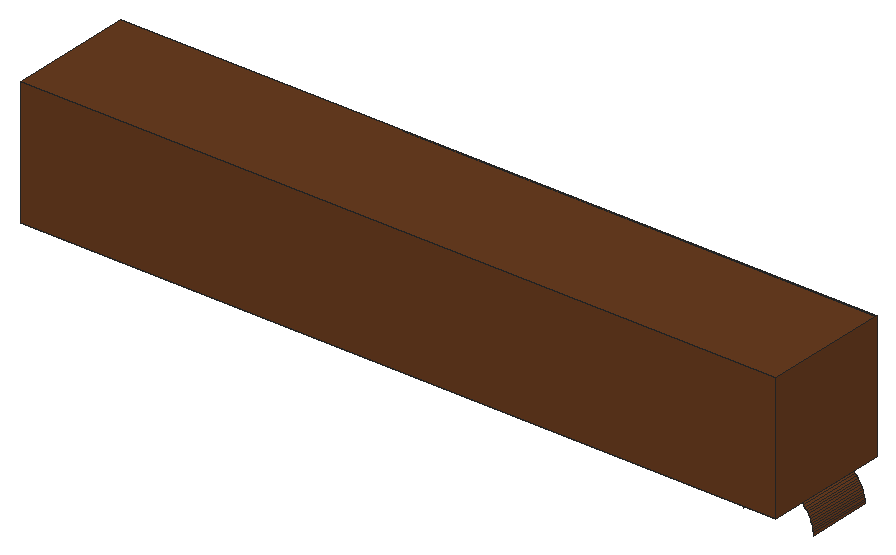
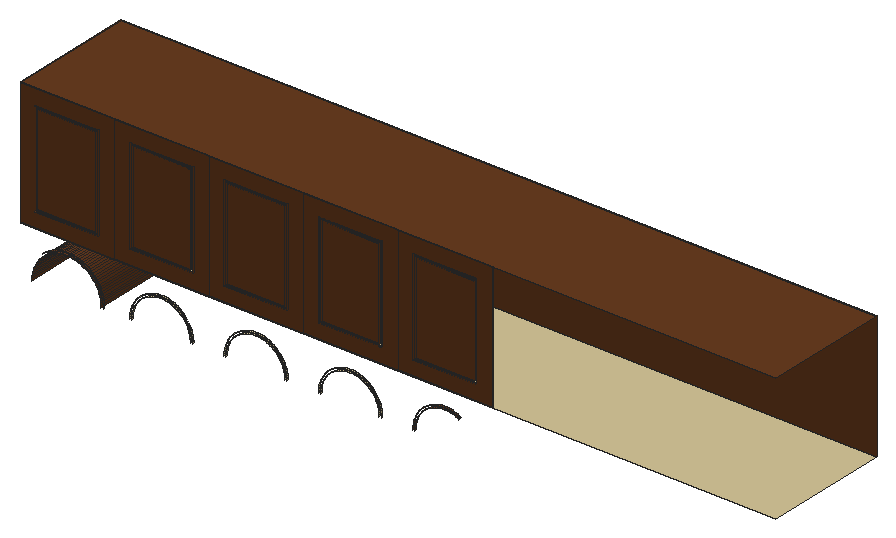
# SketchUp Ruby script. Lengths in inches.
U = 1.inch
M = Sketchup.active_model
def pt(a) = Geom::Point3d.new(a.map { |v| v * U })
def face(e, loops, mat)
  f = e.add_face(loops[0].map { |a| pt(a) })
  loops[1..].each { |l| e.add_face(l.map { |a| pt(a) }).erase! }
  f.material = f.back_material = mat if mat
  f
end
# faces: each face lists its corners as indices into pts; further lists are holes
def faces(e, pts, list, mat = nil) = list.each { |f| face(e, (f[0].is_a?(Array) ? f : [f]).map { |l| l.map { |i| pts[i] } }, mat) }
# xy, xz, yz: faces in a plane at the given z, y or x. An outline is a flat list of corners, or four numbers for a rectangle; further outlines are holes
def ring(l) = l.size == 4 ? [[l[0], l[1]], [l[2], l[1]], [l[2], l[3]], [l[0], l[3]]] : l.each_slice(2).to_a
def flat(e, list, mat, &to3) = list.each { |f| face(e, (f[0].is_a?(Array) ? f : [f]).map { |l| ring(l).map { |u, v| to3.(u, v) } }, mat) }
def xy(e, z, list, mat = nil) = flat(e, list, mat) { |x, y| [x, y, z] }
def xz(e, y, list, mat = nil) = flat(e, list, mat) { |x, z| [x, y, z] }
def yz(e, x, list, mat = nil) = flat(e, list, mat) { |y, z| [x, y, z] }
def lines(e, pts, list) = list.each { |a, b| e.add_line(pt(pts[a]), pt(pts[b])) }
# prism: a flat outline (further loops are holes) pulled along v
def prism(e, loops, v, mat = nil)
  f = face(e, loops, mat); d = Geom::Vector3d.new(v.map { |x| x * U })
  f.pushpull(f.normal.samedirection?(d) ? d.length : -d.length)
end
def box(e, o, s, mat = nil) = prism(e, [[o, [o[0] + s[0], o[1], o[2]], [o[0] + s[0], o[1] + s[1], o[2]], [o[0], o[1] + s[1], o[2]]]], [0, 0, s[2]], mat)
def at(x, y, z, deg = 0) = Geom::Transformation.translation(pt([x, y, z])) * Geom::Transformation.rotation(ORIGIN, Z_AXIS, deg.degrees)
def axes(o, x, y, z) = Geom::Transformation.new([*x, 0, *y, 0, *z, 0, *pt(o).to_a, 1])
def part(name) = M.definitions.add(name)
# library, detail: a bought-in or finely detailed component or shape, given as its bounding box
def library(name, o, s) = part(name).tap { |d| box(d.entities, o, s) }
def detail(e, o, s) = box(e.add_group.entities, o, s)
def put(e, d, t, mat = nil) = e.add_instance(d, t).tap { |i| i.material = mat if mat }
def group(e, t, mat = nil) = e.add_group.tap { |g| g.transformation = t; g.material = mat if mat }.entities
root = M.entities
M.materials.add("138_plaster painted wall texture-seamless").color = [214, 198, 153]
M.materials.add("[0137_Black]").color = [0, 0, 0]
M.materials.add("[Wood Veneer 01]").color = [104, 60, 32]
xy(root,88,[[24,0,168,24]],"138_plaster painted wall texture-seamless")
xy(root,91,[[81,24,93,24.2],[99,24,111,24.2],[117,24,129,24.2],[135,24,147,24.2],[153,24,165,24.2]],"[Wood Veneer 01]")
xy(root,91.4,[[81.4,24,92.6,24.2],[99.4,24,110.6,24.2],[117.4,24,128.6,24.2],[135.4,24,146.6,24.2],[153.4,24,164.6,24.2]],"[Wood Veneer 01]")
xy(root,108.6,[[81.4,24,92.6,24.2],[99.4,24,110.6,24.2],[117.4,24,128.6,24.2],[135.4,24,146.6,24.2],[153.4,24,164.6,24.2]],"[Wood Veneer 01]")
xy(root,109,[[81,24,93,24.2],[99,24,111,24.2],[117,24,129,24.2],[135,24,147,24.2],[153,24,165,24.2]],"[Wood Veneer 01]")
xy(root,112,[[24,0,168,24]],"[Wood Veneer 01]")
xz(root,0,[[24,88,168,112]],"[Wood Veneer 01]")
xz(root,24,[[[78,88,96,112],[78.1,88.1,95.9,111.9]],[[96,88,114,112],[96.1,88.1,113.9,111.9]],[[114,88,132,112],[114.1,88.1,131.9,111.9]],[[132,88,150,112],[132.1,88.1,149.9,111.9]],[[150,88,168,112],[150.1,88.1,167.9,111.9]]],"[0137_Black]")
xz(root,24,[[[78.1,88.1,95.9,111.9],[81,91,93,109]],[[96.1,88.1,113.9,111.9],[99,91,111,109]],[[114.1,88.1,131.9,111.9],[117,91,129,109]],[[132.1,88.1,149.9,111.9],[135,91,147,109]],[[150.1,88.1,167.9,111.9],[153,91,165,109]],
  [81.4,91.4,92.6,108.6],[99.4,91.4,110.6,108.6],[117.4,91.4,128.6,108.6],[135.4,91.4,146.6,108.6],[153.4,91.4,164.6,108.6]],"[Wood Veneer 01]")
yz(root,92.6,[[24,91.4,24.2,108.6]],"[Wood Veneer 01]")
yz(root,93,[[24,91,24.2,109]],"[Wood Veneer 01]")
yz(root,99,[[24,91,24.2,109]],"[Wood Veneer 01]")
yz(root,99.4,[[24,91.4,24.2,108.6]],"[Wood Veneer 01]")
yz(root,110.6,[[24,91.4,24.2,108.6]],"[Wood Veneer 01]")
yz(root,111,[[24,91,24.2,109]],"[Wood Veneer 01]")
yz(root,117,[[24,91,24.2,109]],"[Wood Veneer 01]")
yz(root,117.4,[[24,91.4,24.2,108.6]],"[Wood Veneer 01]")
yz(root,128.6,[[24,91.4,24.2,108.6]],"[Wood Veneer 01]")
yz(root,129,[[24,91,24.2,109]],"[Wood Veneer 01]")
yz(root,135,[[24,91,24.2,109]],"[Wood Veneer 01]")
yz(root,135.4,[[24,91.4,24.2,108.6]],"[Wood Veneer 01]")
yz(root,146.6,[[24,91.4,24.2,108.6]],"[Wood Veneer 01]")
yz(root,147,[[24,91,24.2,109]],"[Wood Veneer 01]")
yz(root,153,[[24,91,24.2,109]],"[Wood Veneer 01]")
yz(root,153.4,[[24,91.4,24.2,108.6]],"[Wood Veneer 01]")
yz(root,168,[[0,88,24,112]],"[Wood Veneer 01]")
p = [[152.4,12,79],[152.4,24.2,79],[152.41,24.2,79.38],[152.41,12,79.38],[165.59,12,79.38],[165.59,24.2,79.38],
  [165.6,24.2,79],[165.6,12,79],[92.6,24,79],[92.59,24,79.33],[92.59,24.2,79.33],[92.6,24.2,79],
  [92.99,24,79.35],[93,24,79],[93,24.2,79],[92.99,24.2,79.35],[99,24,79],[99.01,24,79.35],
  [99.01,24.2,79.35],[99,24.2,79],[99.41,24,79.33],[99.4,24,79],[99.4,24.2,79],[99.41,24.2,79.33],
  [110.6,24,79],[110.59,24,79.33],[110.59,24.2,79.33],[110.6,24.2,79],[110.99,24,79.35],[111,24,79],
  [111,24.2,79],[110.99,24.2,79.35],[117,24,79],[117.01,24,79.35],[117.01,24.2,79.35],[117,24.2,79],
  [117.41,24,79.33],[117.4,24,79],[117.4,24.2,79],[117.41,24.2,79.33],[128.6,24,79],[128.59,24,79.33],
  [128.59,24.2,79.33],[128.6,24.2,79],[128.99,24,79.35],[129,24,79],[129,24.2,79],[128.99,24.2,79.35],
  [135,24,79],[135.01,24,79.35],[135.01,24.2,79.35],[135,24.2,79],[135.41,24,79.33],[135.4,24,79],
  [135.4,24.2,79],[135.41,24.2,79.33],[146.6,24,79],[146.59,24,79.33],[146.59,24.2,79.33],[146.6,24.2,79],
  [146.99,24,79.35],[147,24,79],[147,24.2,79],[146.99,24.2,79.35],[152,24,79],[152.01,24,79.41],
  [152.01,24.2,79.41],[152,24.2,79],[92.5625,24,79.65],[92.5625,24.2,79.65],[92.96,24,79.7],[92.96,24.2,79.7],
  [99.04,24,79.7],[99.04,24.2,79.7],[99.4375,24,79.65],[99.4375,24.2,79.65],[110.5625,24,79.65],[110.5625,24.2,79.65],
  [110.96,24,79.7],[110.96,24.2,79.7],[117.04,24,79.7],[117.04,24.2,79.7],[117.4375,24,79.65],[117.4375,24.2,79.65],
  [128.5625,24,79.65],[128.5625,24.2,79.65],[128.96,24,79.7],[128.96,24.2,79.7],[135.04,24,79.7],[135.04,24.2,79.7],
  [135.4375,24,79.65],[135.4375,24.2,79.65],[146.5625,24,79.65],[146.5625,24.2,79.65],[146.96,24,79.7],[146.96,24.2,79.7],
  [152.44,24.2,79.77],[152.44,12,79.77],[165.56,12,79.77],[165.56,24.2,79.77],[152.05,24,79.8125],[152.05,24.2,79.8125],
  [92.51,24,79.97],[92.51,24.2,79.97],[92.91,24,80.04],[92.91,24.2,80.04],[99.09,24,80.04],[99.09,24.2,80.04],
  [99.49,24,79.97],[99.49,24.2,79.97],[110.51,24,79.97],[110.51,24.2,79.97],[110.91,24,80.04],[110.91,24.2,80.04],
  [117.09,24,80.04],[117.09,24.2,80.04],[117.49,24,79.97],[117.49,24.2,79.97],[128.51,24,79.97],[128.51,24.2,79.97],
  [128.91,24,80.04],[128.91,24.2,80.04],[135.09,24,80.04],[135.09,24.2,80.04],[135.49,24,79.97],[135.49,24.2,79.97],
  [146.51,24,79.97],[146.51,24.2,79.97],[146.91,24,80.04],[146.91,24.2,80.04],[152.5,24.2,80.15],[152.5,12,80.15],
  [165.5,12,80.15],[165.5,24.2,80.15],[152.11,24,80.22],[152.11,24.2,80.22],[92.45,24,80.29],[92.45,24.2,80.29],
  [92.84,24,80.38],[92.84,24.2,80.38],[99.16,24,80.38],[99.16,24.2,80.38],[99.55,24,80.29],[99.55,24.2,80.29],
  [110.45,24,80.29],[110.45,24.2,80.29],[110.84,24,80.38],[110.84,24.2,80.38],[117.16,24,80.38],[117.16,24.2,80.38],
  [117.55,24,80.29],[117.55,24.2,80.29],[128.45,24,80.29],[128.45,24.2,80.29],[128.84,24,80.38],[128.84,24.2,80.38],
  [135.16,24,80.38],[135.16,24.2,80.38],[135.55,24,80.29],[135.55,24.2,80.29],[146.45,24,80.29],[146.45,24.2,80.29],
  [146.84,24,80.38],[146.84,24.2,80.38],[152.58,24.2,80.52],[152.58,12,80.52],[165.42,12,80.52],[165.42,24.2,80.52],
  [152.1875,24,80.61],[152.1875,24.2,80.61],[92.36,24,80.61],[92.36,24.2,80.61],[99.64,24,80.61],[99.64,24.2,80.61],
  [110.36,24,80.61],[110.36,24.2,80.61],[117.64,24,80.61],[117.64,24.2,80.61],[128.36,24,80.61],[128.36,24.2,80.61],
  [135.64,24,80.61],[135.64,24.2,80.61],[146.36,24,80.61],[146.36,24.2,80.61],[92.75,24,80.72],[92.75,24.2,80.72],
  [99.25,24,80.72],[99.25,24.2,80.72],[110.75,24,80.72],[110.75,24.2,80.72],[117.25,24,80.72],[117.25,24.2,80.72],
  [128.75,24,80.72],[128.75,24.2,80.72],[135.25,24,80.72],[135.25,24.2,80.72],[146.75,24,80.72],[146.75,24.2,80.72],
  [152.68,24.2,80.89],[152.68,12,80.89],[165.32,12,80.89],[165.32,24.2,80.89],[92.26,24,80.92],[92.26,24.2,80.92],
  [99.74,24,80.92],[99.74,24.2,80.92],[110.26,24,80.92],[110.26,24.2,80.92],[117.74,24,80.92],[117.74,24.2,80.92],
  [128.26,24,80.92],[128.26,24.2,80.92],[135.74,24,80.92],[135.74,24.2,80.92],[146.26,24,80.92],[146.26,24.2,80.92],
  [152.29,24,81.01],[152.29,24.2,81.01],[92.64,24,81.05],[92.64,24.2,81.05],[99.36,24,81.05],[99.36,24.2,81.05],
  [110.64,24,81.05],[110.64,24.2,81.05],[117.36,24,81.05],[117.36,24.2,81.05],[128.64,24,81.05],[128.64,24.2,81.05],
  [135.36,24,81.05],[135.36,24.2,81.05],[146.64,24,81.05],[146.64,24.2,81.05],[152.8,24.2,81.26],[152.8,12,81.26],
  [165.2,12,81.26],[165.2,24.2,81.26],[92.14,24,81.22],[92.14,24.2,81.22],[99.86,24,81.22],[99.86,24.2,81.22],
  [110.14,24,81.22],[110.14,24.2,81.22],[117.86,24,81.22],[117.86,24.2,81.22],[128.14,24,81.22],[128.14,24.2,81.22],
  [135.86,24,81.22],[135.86,24.2,81.22],[146.14,24,81.22],[146.14,24.2,81.22],[152.42,24,81.39],[152.42,24.2,81.39],
  [92.51,24,81.375],[92.51,24.2,81.375],[99.49,24,81.375],[99.49,24.2,81.375],[110.51,24,81.375],[110.51,24.2,81.375],
  [117.49,24,81.375],[117.49,24.2,81.375],[128.51,24,81.375],[128.51,24.2,81.375],[135.49,24,81.375],[135.49,24.2,81.375],
  [146.51,24,81.375],[146.51,24.2,81.375],[92,24,81.51],[92,24.2,81.51],[100,24,81.51],[100,24.2,81.51],
  [110,24,81.51],[110,24.2,81.51],[118,24,81.51],[118,24.2,81.51],[128,24,81.51],[128,24.2,81.51],
  [136,24,81.51],[136,24.2,81.51],[146,24,81.51],[146,24.2,81.51],[152.94,24.2,81.61],[152.94,12,81.61],
  [165.06,12,81.61],[165.06,24.2,81.61],[92.36,24,81.69],[92.36,24.2,81.69],[99.64,24,81.69],[99.64,24.2,81.69],
  [110.36,24,81.69],[110.36,24.2,81.69],[117.64,24,81.69],[117.64,24.2,81.69],[128.36,24,81.69],[128.36,24.2,81.69],
  [135.64,24,81.69],[135.64,24.2,81.69],[146.36,24,81.69],[146.36,24.2,81.69],[152.57,24,81.77],[152.57,24.2,81.77],
  [91.85,24,81.8],[91.85,24.2,81.8],[100.15,24,81.8],[100.15,24.2,81.8],[109.85,24,81.8],[109.85,24.2,81.8],
  [118.15,24,81.8],[118.15,24.2,81.8],[127.85,24,81.8],[127.85,24.2,81.8],[136.15,24,81.8],[136.15,24.2,81.8],
  [145.85,24,81.8],[145.85,24.2,81.8],[153.1,24.2,81.96],[153.1,12,81.96],[164.9,12,81.96],[164.9,24.2,81.96],
  [92.2,24,82],[92.2,24.2,82],[99.8,24,82],[99.8,24.2,82],[110.2,24,82],[110.2,24.2,82],
  [117.8,24,82],[117.8,24.2,82],[128.2,24,82],[128.2,24.2,82],[135.8,24,82],[135.8,24.2,82],
  [146.2,24,82],[146.2,24.2,82],[91.68,24,82.08],[91.68,24.2,82.08],[100.32,24,82.08],[100.32,24.2,82.08],
  [109.68,24,82.08],[109.68,24.2,82.08],[118.32,24,82.08],[118.32,24.2,82.08],[127.68,24,82.08],[127.68,24.2,82.08],
  [136.32,24,82.08],[136.32,24.2,82.08],[145.68,24,82.08],[145.68,24.2,82.08],[152.74,24,82.14],[152.74,24.2,82.14],
  [153.28,24.2,82.3],[153.28,12,82.3],[164.72,12,82.3],[164.72,24.2,82.3],[92.01,24,82.3],[92.01,24.2,82.3],
  [99.99,24,82.3],[99.99,24.2,82.3],[110.01,24,82.3],[110.01,24.2,82.3],[117.99,24,82.3],[117.99,24.2,82.3],
  [128.01,24,82.3],[128.01,24.2,82.3],[135.99,24,82.3],[135.99,24.2,82.3],[146.01,24,82.3],[146.01,24.2,82.3],
  [91.49,24,82.34],[91.49,24.2,82.34],[100.51,24,82.34],[100.51,24.2,82.34],[109.49,24,82.34],[109.49,24.2,82.34],
  [118.51,24,82.34],[118.51,24.2,82.34],[127.49,24,82.34],[127.49,24.2,82.34],[136.51,24,82.34],[136.51,24.2,82.34],
  [145.49,24,82.34],[145.49,24.2,82.34],[152.9375,24,82.5],[152.9375,24.2,82.5],[153.49,24.2,82.625],[153.49,12,82.625],
  [164.51,12,82.625],[164.51,24.2,82.625],[91.29,24,82.6],[91.29,24.2,82.6],[91.8125,24,82.58],[91.8125,24.2,82.58],
  [100.1875,24,82.58],[100.1875,24.2,82.58],[100.71,24,82.6],[100.71,24.2,82.6],[109.29,24,82.6],[109.29,24.2,82.6],
  [109.8125,24,82.58],[109.8125,24.2,82.58],[118.1875,24,82.58],[118.1875,24.2,82.58],[118.71,24,82.6],[118.71,24.2,82.6],
  [127.29,24,82.6],[127.29,24.2,82.6],[127.8125,24,82.58],[127.8125,24.2,82.58],[136.1875,24,82.58],[136.1875,24.2,82.58],
  [136.71,24,82.6],[136.71,24.2,82.6],[145.29,24,82.6],[145.29,24.2,82.6],[145.8125,24,82.58],[145.8125,24.2,82.58],
  [153.15,24,82.85],[153.15,24.2,82.85],[153.71,24.2,82.94],[153.71,12,82.94],[164.29,12,82.94],[164.29,24.2,82.94],
  [91.07,24,82.84],[91.07,24.2,82.84],[91.6,24,82.86],[91.6,24.2,82.86],[100.4,24,82.86],[100.4,24.2,82.86],
  [100.93,24,82.84],[100.93,24.2,82.84],[109.07,24,82.84],[109.07,24.2,82.84],[109.6,24,82.86],[109.6,24.2,82.86],
  [118.4,24,82.86],[118.4,24.2,82.86],[118.93,24,82.84],[118.93,24.2,82.84],[127.07,24,82.84],[127.07,24.2,82.84],
  [127.6,24,82.86],[127.6,24.2,82.86],[136.4,24,82.86],[136.4,24.2,82.86],[136.93,24,82.84],[136.93,24.2,82.84],
  [145.07,24,82.84],[145.07,24.2,82.84],[145.6,24,82.86],[145.6,24.2,82.86],[90.84,24,83.07],[90.84,24.2,83.07],
  [101.16,24,83.07],[101.16,24.2,83.07],[108.84,24,83.07],[108.84,24.2,83.07],[119.16,24,83.07],[119.16,24.2,83.07],
  [126.84,24,83.07],[126.84,24.2,83.07],[137.16,24,83.07],[137.16,24.2,83.07],[144.84,24,83.07],[144.84,24.2,83.07],
  [153.39,24,83.18],[153.39,24.2,83.18],[153.94,24.2,83.24],[153.94,12,83.24],[164.06,12,83.24],[164.06,24.2,83.24],
  [91.36,24,83.12],[91.36,24.2,83.12],[100.64,24,83.12],[100.64,24.2,83.12],[109.36,24,83.12],[109.36,24.2,83.12],
  [118.64,24,83.12],[118.64,24.2,83.12],[127.36,24,83.12],[127.36,24.2,83.12],[136.64,24,83.12],[136.64,24.2,83.12],
  [145.36,24,83.12],[145.36,24.2,83.12],[90.6,24,83.29],[90.6,24.2,83.29],[91.12,24,83.36],[91.12,24.2,83.36],
  [100.88,24,83.36],[100.88,24.2,83.36],[101.4,24,83.29],[101.4,24.2,83.29],[108.6,24,83.29],[108.6,24.2,83.29],
  [109.12,24,83.36],[109.12,24.2,83.36],[118.88,24,83.36],[118.88,24.2,83.36],[119.4,24,83.29],[119.4,24.2,83.29],
  [126.6,24,83.29],[126.6,24.2,83.29],[127.12,24,83.36],[127.12,24.2,83.36],[136.88,24,83.36],[136.88,24.2,83.36],
  [137.4,24,83.29],[137.4,24.2,83.29],[144.6,24,83.29],[144.6,24.2,83.29],[145.12,24,83.36],[145.12,24.2,83.36],
  [154.2,24.2,83.53],[154.2,12,83.53],[163.8,12,83.53],[163.8,24.2,83.53],[153.64,24,83.5],[153.64,24.2,83.5],
  [90.34,24,83.49],[90.34,24.2,83.49],[101.66,24,83.49],[101.66,24.2,83.49],[108.34,24,83.49],[108.34,24.2,83.49],
  [119.66,24,83.49],[119.66,24.2,83.49],[126.34,24,83.49],[126.34,24.2,83.49],[137.66,24,83.49],[137.66,24.2,83.49],
  [144.34,24,83.49],[144.34,24.2,83.49],[90.86,24,83.6],[90.86,24.2,83.6],[101.14,24,83.6],[101.14,24.2,83.6],
  [108.86,24,83.6],[108.86,24.2,83.6],[119.14,24,83.6],[119.14,24.2,83.6],[126.86,24,83.6],[126.86,24.2,83.6],
  [137.14,24,83.6],[137.14,24.2,83.6],[144.86,24,83.6],[144.86,24.2,83.6],[154.47,24.2,83.8],[154.47,12,83.8],
  [163.53,12,83.8],[163.53,24.2,83.8],[90.08,24,83.68],[90.08,24.2,83.68],[101.92,24,83.68],[101.92,24.2,83.68],
  [108.08,24,83.68],[108.08,24.2,83.68],[119.92,24,83.68],[119.92,24.2,83.68],[126.08,24,83.68],[126.08,24.2,83.68],
  [137.92,24,83.68],[137.92,24.2,83.68],[144.08,24,83.68],[144.08,24.2,83.68],[153.91,24,83.8],[153.91,24.2,83.8],
  [90.58,24,83.8125],[90.58,24.2,83.8125],[101.42,24,83.8125],[101.42,24.2,83.8125],[108.58,24,83.8125],[108.58,24.2,83.8125],
  [119.42,24,83.8125],[119.42,24.2,83.8125],[126.58,24,83.8125],[126.58,24.2,83.8125],[137.42,24,83.8125],[137.42,24.2,83.8125],
  [144.58,24,83.8125],[144.58,24.2,83.8125],[89.8,24,83.85],[89.8,24.2,83.85],[102.2,24,83.85],[102.2,24.2,83.85],
  [107.8,24,83.85],[107.8,24.2,83.85],[120.2,24,83.85],[120.2,24.2,83.85],[125.8,24,83.85],[125.8,24.2,83.85],
  [138.2,24,83.85],[138.2,24.2,83.85],[143.8,24,83.85],[143.8,24.2,83.85],[154.76,24.2,84.06],[154.76,12,84.06],
  [163.24,12,84.06],[163.24,24.2,84.06],[84.49,24,84],[84.2,24,83.85],[84.2,24.2,83.85],[84.49,24.2,84],
  [89.51,24,84],[89.51,24.2,84],[90.3,24,84.01],[90.3,24.2,84.01],[101.7,24,84.01],[101.7,24.2,84.01],
  [102.49,24,84],[102.49,24.2,84],[107.51,24,84],[107.51,24.2,84],[108.3,24,84.01],[108.3,24.2,84.01],
  [119.7,24,84.01],[119.7,24.2,84.01],[120.49,24,84],[120.49,24.2,84],[125.51,24,84],[125.51,24.2,84],
  [126.3,24,84.01],[126.3,24.2,84.01],[137.7,24,84.01],[137.7,24.2,84.01],[138.49,24,84],[138.49,24.2,84],
  [143.51,24,84],[143.51,24.2,84],[144.3,24,84.01],[144.3,24.2,84.01],[154.2,24,84.09],[154.2,24.2,84.09],
  [84.78,24,84.14],[84.78,24.2,84.14],[89.22,24,84.14],[89.22,24.2,84.14],[90,24,84.2],[90,24.2,84.2],
  [102,24,84.2],[102,24.2,84.2],[102.78,24,84.14],[102.78,24.2,84.14],[107.22,24,84.14],[107.22,24.2,84.14],
  [108,24,84.2],[108,24.2,84.2],[120,24,84.2],[120,24.2,84.2],[120.78,24,84.14],[120.78,24.2,84.14],
  [125.22,24,84.14],[125.22,24.2,84.14],[126,24,84.2],[126,24.2,84.2],[138,24,84.2],[138,24.2,84.2],
  [138.78,24,84.14],[138.78,24.2,84.14],[143.22,24,84.14],[143.22,24.2,84.14],[144,24,84.2],[144,24.2,84.2],
  [155.06,24.2,84.29],[155.06,12,84.29],[162.94,12,84.29],[162.94,24.2,84.29],[85.08,24,84.26],[85.08,24.2,84.26],
  [88.92,24,84.26],[88.92,24.2,84.26],[103.08,24,84.26],[103.08,24.2,84.26],[106.92,24,84.26],[106.92,24.2,84.26],
  [121.08,24,84.26],[121.08,24.2,84.26],[124.92,24,84.26],[124.92,24.2,84.26],[139.08,24,84.26],[139.08,24.2,84.26],
  [142.92,24,84.26],[142.92,24.2,84.26],[154.5,24,84.36],[154.5,24.2,84.36],[163.5,24,84.36],[163.8,24,84.09],
  [163.8,24.2,84.09],[163.5,24.2,84.36],[84,24,84.2],[84.31,24,84.36],[84.31,24.2,84.36],[84,24.2,84.2],
  [89.69,24,84.36],[89.69,24.2,84.36],[102.31,24,84.36],[102.31,24.2,84.36],[107.69,24,84.36],[107.69,24.2,84.36],
  [120.31,24,84.36],[120.31,24.2,84.36],[125.69,24,84.36],[125.69,24.2,84.36],[138.31,24,84.36],[138.31,24.2,84.36],
  [143.69,24,84.36],[143.69,24.2,84.36],[155.375,24.2,84.51],[155.375,12,84.51],[162.625,12,84.51],[162.625,24.2,84.51],
  [85.39,24,84.36],[85.39,24.2,84.36],[88.61,24,84.36],[88.61,24.2,84.36],[103.39,24,84.36],[103.39,24.2,84.36],
  [106.61,24,84.36],[106.61,24.2,84.36],[121.39,24,84.36],[121.39,24.2,84.36],[124.61,24,84.36],[124.61,24.2,84.36],
  [139.39,24,84.36],[139.39,24.2,84.36],[142.61,24,84.36],[142.61,24.2,84.36],[84.625,24,84.51],[84.625,24.2,84.51],
  [85.71,24,84.45],[85.71,24.2,84.45],[86.03,24,84.51],[86.03,24.2,84.51],[88.29,24,84.45],[87.97,24,84.51],
  [87.97,24.2,84.51],[88.29,24.2,84.45],[89.375,24,84.51],[89.375,24.2,84.51],[102.625,24,84.51],[102.625,24.2,84.51],
  [103.71,24,84.45],[103.71,24.2,84.45],[104.03,24,84.51],[104.03,24.2,84.51],[106.29,24,84.45],[105.97,24,84.51],
  [105.97,24.2,84.51],[106.29,24.2,84.45],[107.375,24,84.51],[107.375,24.2,84.51],[120.625,24,84.51],[120.625,24.2,84.51],
  [121.71,24,84.45],[121.71,24.2,84.45],[122.03,24,84.51],[122.03,24.2,84.51],[124.29,24,84.45],[123.97,24,84.51],
  [123.97,24.2,84.51],[124.29,24.2,84.45],[125.375,24,84.51],[125.375,24.2,84.51],[138.625,24,84.51],[138.625,24.2,84.51],
  [139.71,24,84.45],[139.71,24.2,84.45],[140.03,24,84.51],[140.03,24.2,84.51],[142.29,24,84.45],[141.97,24,84.51],
  [141.97,24.2,84.51],[142.29,24.2,84.45],[143.375,24,84.51],[143.375,24.2,84.51],[154.82,24,84.61],[154.82,24.2,84.61],
  [163.18,24,84.61],[163.18,24.2,84.61],[155.7,24.2,84.72],[155.7,12,84.72],[162.3,12,84.72],[162.3,24.2,84.72],
  [84.95,24,84.64],[84.95,24.2,84.64],[86.35,24,84.5625],[86.35,24.2,84.5625],[87.65,24,84.5625],[87.65,24.2,84.5625],
  [89.05,24,84.64],[89.05,24.2,84.64],[102.95,24,84.64],[102.95,24.2,84.64],[104.35,24,84.5625],[104.35,24.2,84.5625],
  [105.65,24,84.5625],[105.65,24.2,84.5625],[107.05,24,84.64],[107.05,24.2,84.64],[120.95,24,84.64],[120.95,24.2,84.64],
  [122.35,24,84.5625],[122.35,24.2,84.5625],[123.65,24,84.5625],[123.65,24.2,84.5625],[125.05,24,84.64],[125.05,24.2,84.64],
  [138.95,24,84.64],[138.95,24.2,84.64],[140.35,24,84.5625],[140.35,24.2,84.5625],[141.65,24,84.5625],[141.65,24.2,84.5625],
  [143.05,24,84.64],[143.05,24.2,84.64],[85.28,24,84.75],[85.28,24.2,84.75],[86.67,24,84.59],[86.67,24.2,84.59],
  [87,24,84.6],[87,24.2,84.6],[87.33,24,84.59],[87.33,24.2,84.59],[88.72,24,84.75],[88.72,24.2,84.75],
  [103.28,24,84.75],[103.28,24.2,84.75],[104.67,24,84.59],[104.67,24.2,84.59],[105,24,84.6],[105,24.2,84.6],
  [105.33,24,84.59],[105.33,24.2,84.59],[106.72,24,84.75],[106.72,24.2,84.75],[121.28,24,84.75],[121.28,24.2,84.75],
  [122.67,24,84.59],[122.67,24.2,84.59],[123,24,84.6],[123,24.2,84.6],[123.33,24,84.59],[123.33,24.2,84.59],
  [124.72,24,84.75],[124.72,24.2,84.75],[139.28,24,84.75],[139.28,24.2,84.75],[140.67,24,84.59],[140.67,24.2,84.59],
  [141,24,84.6],[141,24.2,84.6],[141.33,24,84.59],[141.33,24.2,84.59],[142.72,24,84.75],[142.72,24.2,84.75],
  [155.15,24,84.85],[155.15,24.2,84.85],[162.85,24,84.85],[162.85,24.2,84.85],[156.04,24.2,84.9],[156.04,12,84.9],
  [161.96,12,84.9],[161.96,24.2,84.9],[85.62,24,84.84],[85.62,24.2,84.84],[88.38,24,84.84],[88.38,24.2,84.84],
  [103.62,24,84.84],[103.62,24.2,84.84],[106.38,24,84.84],[106.38,24.2,84.84],[121.62,24,84.84],[121.62,24.2,84.84],
  [124.38,24,84.84],[124.38,24.2,84.84],[139.62,24,84.84],[139.62,24.2,84.84],[142.38,24,84.84],[142.38,24.2,84.84],
  [85.96,24,84.91],[85.96,24.2,84.91],[88.04,24,84.91],[88.04,24.2,84.91],[103.96,24,84.91],[103.96,24.2,84.91],
  [106.04,24,84.91],[106.04,24.2,84.91],[121.96,24,84.91],[121.96,24.2,84.91],[124.04,24,84.91],[124.04,24.2,84.91],
  [139.96,24,84.91],[139.96,24.2,84.91],[142.04,24,84.91],[142.04,24.2,84.91],[155.5,24,85.0625],[155.5,24.2,85.0625],
  [162.5,24,85.0625],[162.5,24.2,85.0625],[156.39,24.2,85.06],[156.39,12,85.06],[161.61,12,85.06],[161.61,24.2,85.06],
  [86.3,24,84.96],[86.3,24.2,84.96],[87.7,24,84.96],[87.7,24.2,84.96],[104.3,24,84.96],[104.3,24.2,84.96],
  [105.7,24,84.96],[105.7,24.2,84.96],[122.3,24,84.96],[122.3,24.2,84.96],[123.7,24,84.96],[123.7,24.2,84.96],
  [140.3,24,84.96],[140.3,24.2,84.96],[141.7,24,84.96],[141.7,24.2,84.96],[86.65,24,84.99],[86.65,24.2,84.99],
  [87,24,85],[87,24.2,85],[87.35,24,84.99],[87.35,24.2,84.99],[104.65,24,84.99],[104.65,24.2,84.99],
  [105,24,85],[105,24.2,85],[105.35,24,84.99],[105.35,24.2,84.99],[122.65,24,84.99],[122.65,24.2,84.99],
  [123,24,85],[123,24.2,85],[123.35,24,84.99],[123.35,24.2,84.99],[140.65,24,84.99],[140.65,24.2,84.99],
  [141,24,85],[141,24.2,85],[141.35,24,84.99],[141.35,24.2,84.99],[156.74,24.2,85.2],[156.74,12,85.2],
  [161.26,12,85.2],[161.26,24.2,85.2],[155.86,24,85.26],[155.86,24.2,85.26],[162.14,24,85.26],[162.14,24.2,85.26],
  [157.11,24.2,85.32],[157.11,12,85.32],[160.89,12,85.32],[160.89,24.2,85.32],[157.48,24.2,85.42],[157.48,12,85.42],
  [160.52,12,85.42],[160.52,24.2,85.42],[156.23,24,85.43],[156.23,24.2,85.43],[161.77,24,85.43],[161.77,24.2,85.43],
  [157.85,24.2,85.5],[157.85,12,85.5],[160.15,12,85.5],[160.15,24.2,85.5],[156.61,24,85.58],[156.61,24.2,85.58],
  [161.39,24,85.58],[161.39,24.2,85.58],[158.23,24.2,85.56],[158.23,12,85.56],[159.77,12,85.56],[159.77,24.2,85.56],
  [158.62,24.2,85.59],[158.62,12,85.59],[159,24.2,85.6],[159,12,85.6],[159.38,24.2,85.59],[159.38,12,85.59],
  [156.99,24,85.71],[156.99,24.2,85.71],[161.01,24,85.71],[161.01,24.2,85.71],[157.39,24,85.8125],[157.39,24.2,85.8125],
  [160.61,24,85.8125],[160.61,24.2,85.8125],[157.78,24,85.89],[157.78,24.2,85.89],[160.22,24,85.89],[160.22,24.2,85.89],
  [158.1875,24,85.95],[158.1875,24.2,85.95],[159.8125,24,85.95],[159.8125,24.2,85.95],[158.59,24,85.99],[158.59,24.2,85.99],
  [159,24,86],[159,24.2,86],[159.41,24,85.99],[159.41,24.2,85.99]]
faces(root,p,[[0,1,2,3],[4,5,6,7],[8,9,10,11],[12,13,14,15],[64,65,66,67],[9,68,69,10],[70,12,15,71],[3,2,96,97],
  [98,99,5,4],[65,100,101,66],[68,102,103,69],[104,70,71,105],[97,96,130,131],[132,133,99,98],[100,134,135,101],[102,136,137,103],
  [138,104,105,139],[131,130,164,165],[166,167,133,132],[134,168,169,135],[136,170,171,137],[184,138,139,185],[165,164,198,199],[200,201,167,166],
  [170,202,203,171],[168,216,217,169],[218,184,185,219],[199,198,232,233],[234,235,201,200],[202,236,237,203],[216,250,251,217],[252,218,219,253],
  [236,266,267,237],[233,232,280,281],[282,283,235,234],[284,252,253,285],[250,298,299,251],[266,300,301,267],[281,280,314,315],[316,317,283,282],
  [318,284,285,319],[300,332,333,301],[298,346,347,299],[315,314,348,349],[350,351,317,316],[352,318,319,353],[332,366,367,333],[346,380,381,347],
  [349,348,382,383],[384,385,351,350],[366,386,387,367],[388,352,353,389],[380,414,415,381],[383,382,416,417],[418,419,385,384],[386,420,421,387],
  [422,388,389,423],[420,448,449,421],[414,462,463,415],[417,416,464,465],[466,467,419,418],[468,422,423,469],[448,482,483,449],[484,468,469,485],
  [465,464,510,511],[512,513,467,466],[462,514,515,463],[482,516,517,483],[530,484,485,531],[511,510,544,545],[546,547,513,512],[516,548,549,517],
  [514,562,563,515],[564,530,531,565],[548,578,579,549],[545,544,592,593],[594,595,547,546],[596,597,598,599],[578,600,601,579],[602,564,565,603],
  [562,628,629,563],[630,596,599,631],[600,632,633,601],[634,602,603,635],[593,592,660,661],[662,663,595,594],[664,630,631,665],[632,666,667,633],
  [628,680,681,629],[682,683,684,685],[686,687,688,689],[690,634,635,691],[661,660,704,705],[706,707,663,662],[708,664,665,709],[666,710,711,667],
  [687,724,725,688],[726,708,709,727],[728,726,727,729],[730,731,732,733],[710,730,733,711],[734,690,691,735],[680,772,773,681],[774,682,685,775],
  [705,704,776,777],[778,779,707,706],[724,780,781,725],[782,728,729,783],[731,784,785,732],[786,734,735,787],[780,812,813,781],[814,782,783,815],
  [816,814,815,817],[818,816,817,819],[784,818,819,785],[820,786,787,821],[772,852,853,773],[854,774,775,855],[777,776,856,857],[858,859,779,778],
  [812,860,861,813],[862,820,821,863],[860,876,877,861],[878,862,863,879],[852,892,893,853],[894,854,855,895],[857,856,896,897],[898,899,859,858],
  [876,900,901,877],[902,878,879,903],[900,916,917,901],[916,918,919,917],[918,920,921,919],[920,902,903,921],[897,896,940,941],[942,943,899,898],
  [892,944,945,893],[946,894,895,947],[941,940,948,949],[950,951,943,942],[949,948,952,953],[954,955,951,950],[944,956,957,945],[958,946,947,959],
  [953,952,960,961],[962,963,955,954],[956,964,965,957],[966,958,959,967],[961,960,968,969],[970,971,963,962],[969,968,972,973],[973,972,974,975],
  [975,974,976,977],[977,976,971,970],[964,978,979,965],[980,966,967,981],[978,982,983,979],[984,980,981,985],[982,986,987,983],[988,984,985,989],
  [986,990,991,987],[992,988,989,993],[990,994,995,991],[994,996,997,995],[996,998,999,997],[998,992,993,999]],"[Wood Veneer 01]")
faces(root,p,[[16,17,18,19],[20,21,22,23],[24,25,26,27],[28,29,30,31],[32,33,34,35],[36,37,38,39],[40,41,42,43],[44,45,46,47],
  [48,49,50,51],[52,53,54,55],[56,57,58,59],[60,61,62,63],[17,72,73,18],[74,20,23,75],[25,76,77,26],[78,28,31,79],
  [33,80,81,34],[82,36,39,83],[41,84,85,42],[86,44,47,87],[49,88,89,50],[90,52,55,91],[57,92,93,58],[94,60,63,95],
  [72,106,107,73],[108,74,75,109],[76,110,111,77],[112,78,79,113],[80,114,115,81],[116,82,83,117],[84,118,119,85],[120,86,87,121],
  [88,122,123,89],[124,90,91,125],[92,126,127,93],[128,94,95,129],[106,140,141,107],[142,108,109,143],[110,144,145,111],[146,112,113,147],
  [114,148,149,115],[150,116,117,151],[118,152,153,119],[154,120,121,155],[122,156,157,123],[158,124,125,159],[126,160,161,127],[162,128,129,163],
  [172,142,143,173],[144,174,175,145],[176,150,151,177],[152,178,179,153],[180,158,159,181],[160,182,183,161],[140,186,187,141],[188,146,147,189],
  [148,190,191,149],[192,154,155,193],[156,194,195,157],[196,162,163,197],[204,172,173,205],[174,206,207,175],[208,176,177,209],[178,210,211,179],
  [212,180,181,213],[182,214,215,183],[186,220,221,187],[222,188,189,223],[190,224,225,191],[226,192,193,227],[194,228,229,195],[230,196,197,231],
  [238,204,205,239],[206,240,241,207],[242,208,209,243],[210,244,245,211],[246,212,213,247],[214,248,249,215],[220,254,255,221],[256,222,223,257],
  [224,258,259,225],[260,226,227,261],[228,262,263,229],[264,230,231,265],[268,238,239,269],[240,270,271,241],[272,242,243,273],[244,274,275,245],
  [276,246,247,277],[248,278,279,249],[254,286,287,255],[288,256,257,289],[258,290,291,259],[292,260,261,293],[262,294,295,263],[296,264,265,297],
  [302,268,269,303],[270,304,305,271],[306,272,273,307],[274,308,309,275],[310,276,277,311],[278,312,313,279],[286,320,321,287],[322,288,289,323],
  [290,324,325,291],[326,292,293,327],[294,328,329,295],[330,296,297,331],[334,302,303,335],[304,336,337,305],[338,306,307,339],[308,340,341,309],
  [342,310,311,343],[312,344,345,313],[320,354,355,321],[356,322,323,357],[324,358,359,325],[360,326,327,361],[328,362,363,329],[364,330,331,365],
  [368,334,335,369],[336,370,371,337],[372,338,339,373],[340,374,375,341],[376,342,343,377],[344,378,379,345],[354,390,391,355],[392,368,369,393],
  [370,394,395,371],[396,356,357,397],[358,398,399,359],[400,372,373,401],[374,402,403,375],[404,360,361,405],[362,406,407,363],[408,376,377,409],
  [378,410,411,379],[412,364,365,413],[390,424,425,391],[426,392,393,427],[394,428,429,395],[430,396,397,431],[398,432,433,399],[434,400,401,435],
  [402,436,437,403],[438,404,405,439],[406,440,441,407],[442,408,409,443],[410,444,445,411],[446,412,413,447],[450,426,427,451],[428,452,453,429],
  [454,434,435,455],[436,456,457,437],[458,442,443,459],[444,460,461,445],[424,470,471,425],[472,430,431,473],[432,474,475,433],[476,438,439,477],
  [440,478,479,441],[480,446,447,481],[470,486,487,471],[488,450,451,489],[452,490,491,453],[492,472,473,493],[474,494,495,475],[496,454,455,497],
  [456,498,499,457],[500,476,477,501],[478,502,503,479],[504,458,459,505],[460,506,507,461],[508,480,481,509],[518,488,489,519],[490,520,521,491],
  [522,496,497,523],[498,524,525,499],[526,504,505,527],[506,528,529,507],[486,532,533,487],[534,492,493,535],[494,536,537,495],[538,500,501,539],
  [502,540,541,503],[542,508,509,543],[550,518,519,551],[520,552,553,521],[554,522,523,555],[524,556,557,525],[558,526,527,559],[528,560,561,529],
  [532,566,567,533],[568,534,535,569],[536,570,571,537],[572,538,539,573],[540,574,575,541],[576,542,543,577],[580,550,551,581],[552,582,583,553],
  [584,554,555,585],[556,586,587,557],[588,558,559,589],[560,590,591,561],[566,604,605,567],[606,580,581,607],[582,608,609,583],[610,568,569,611],
  [570,612,613,571],[614,584,585,615],[586,616,617,587],[618,572,573,619],[574,620,621,575],[622,588,589,623],[590,624,625,591],[626,576,577,627],
  [604,636,637,605],[638,606,607,639],[608,640,641,609],[642,610,611,643],[612,644,645,613],[646,614,615,647],[616,648,649,617],[650,618,619,651],
  [620,652,653,621],[654,622,623,655],[624,656,657,625],[658,626,627,659],[668,638,639,669],[640,670,671,641],[672,646,647,673],[648,674,675,649],
  [676,654,655,677],[656,678,679,657],[636,692,693,637],[694,642,643,695],[644,696,697,645],[698,650,651,699],[652,700,701,653],[702,658,659,703],
  [712,668,669,713],[670,714,715,671],[716,672,673,717],[674,718,719,675],[720,676,677,721],[678,722,723,679],[692,736,737,693],[738,712,713,739],
  [740,738,739,741],[742,743,744,745],[714,742,745,715],[746,694,695,747],[696,748,749,697],[750,716,717,751],[752,750,751,753],[754,755,756,757],
  [718,754,757,719],[758,698,699,759],[700,760,761,701],[762,720,721,763],[764,762,763,765],[766,767,768,769],[722,766,769,723],[770,702,703,771],
  [736,788,789,737],[790,740,741,791],[743,792,793,744],[794,746,747,795],[748,796,797,749],[798,752,753,799],[755,800,801,756],[802,758,759,803],
  [760,804,805,761],[806,764,765,807],[767,808,809,768],[810,770,771,811],[788,822,823,789],[824,790,791,825],[826,824,825,827],[828,826,827,829],
  [792,828,829,793],[830,794,795,831],[796,832,833,797],[834,798,799,835],[836,834,835,837],[838,836,837,839],[800,838,839,801],[840,802,803,841],
  [804,842,843,805],[844,806,807,845],[846,844,845,847],[848,846,847,849],[808,848,849,809],[850,810,811,851],[822,864,865,823],[866,830,831,867],
  [832,868,869,833],[870,840,841,871],[842,872,873,843],[874,850,851,875],[864,880,881,865],[882,866,867,883],[868,884,885,869],[886,870,871,887],
  [872,888,889,873],[890,874,875,891],[880,904,905,881],[906,882,883,907],[884,908,909,885],[910,886,887,911],[888,912,913,889],[914,890,891,915],
  [904,922,923,905],[922,924,925,923],[924,926,927,925],[926,906,907,927],[908,928,929,909],[928,930,931,929],[930,932,933,931],[932,910,911,933],
  [912,934,935,913],[934,936,937,935],[936,938,939,937],[938,914,915,939]],"138_plaster painted wall texture-seamless")
